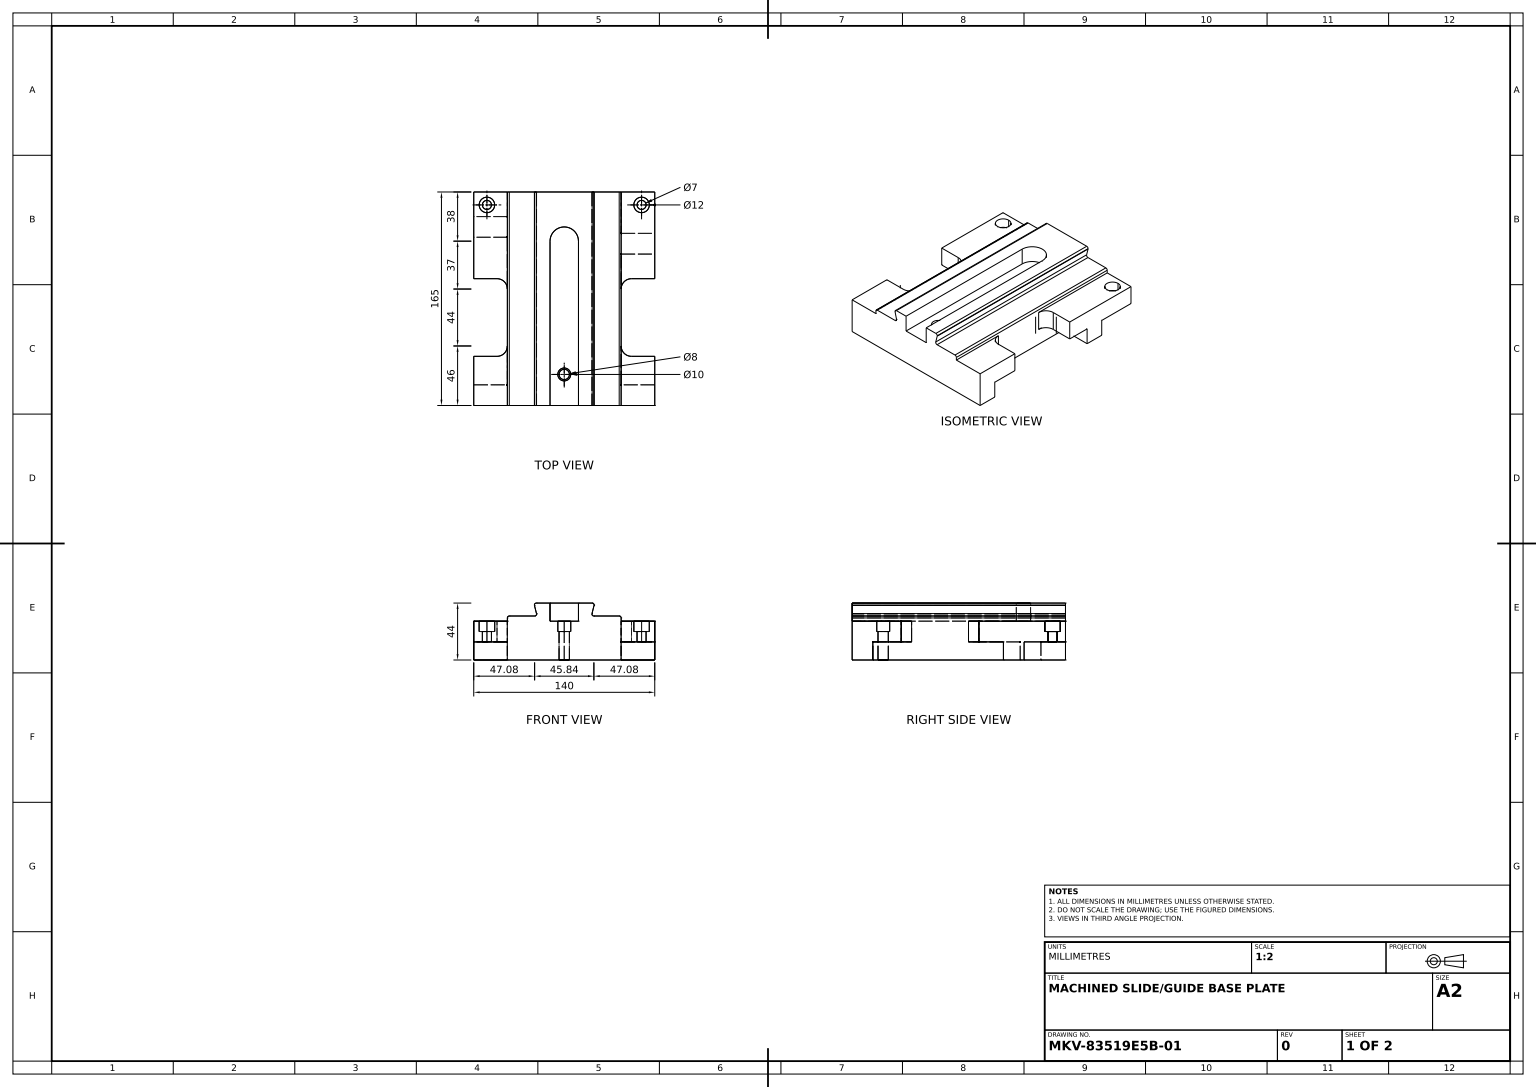
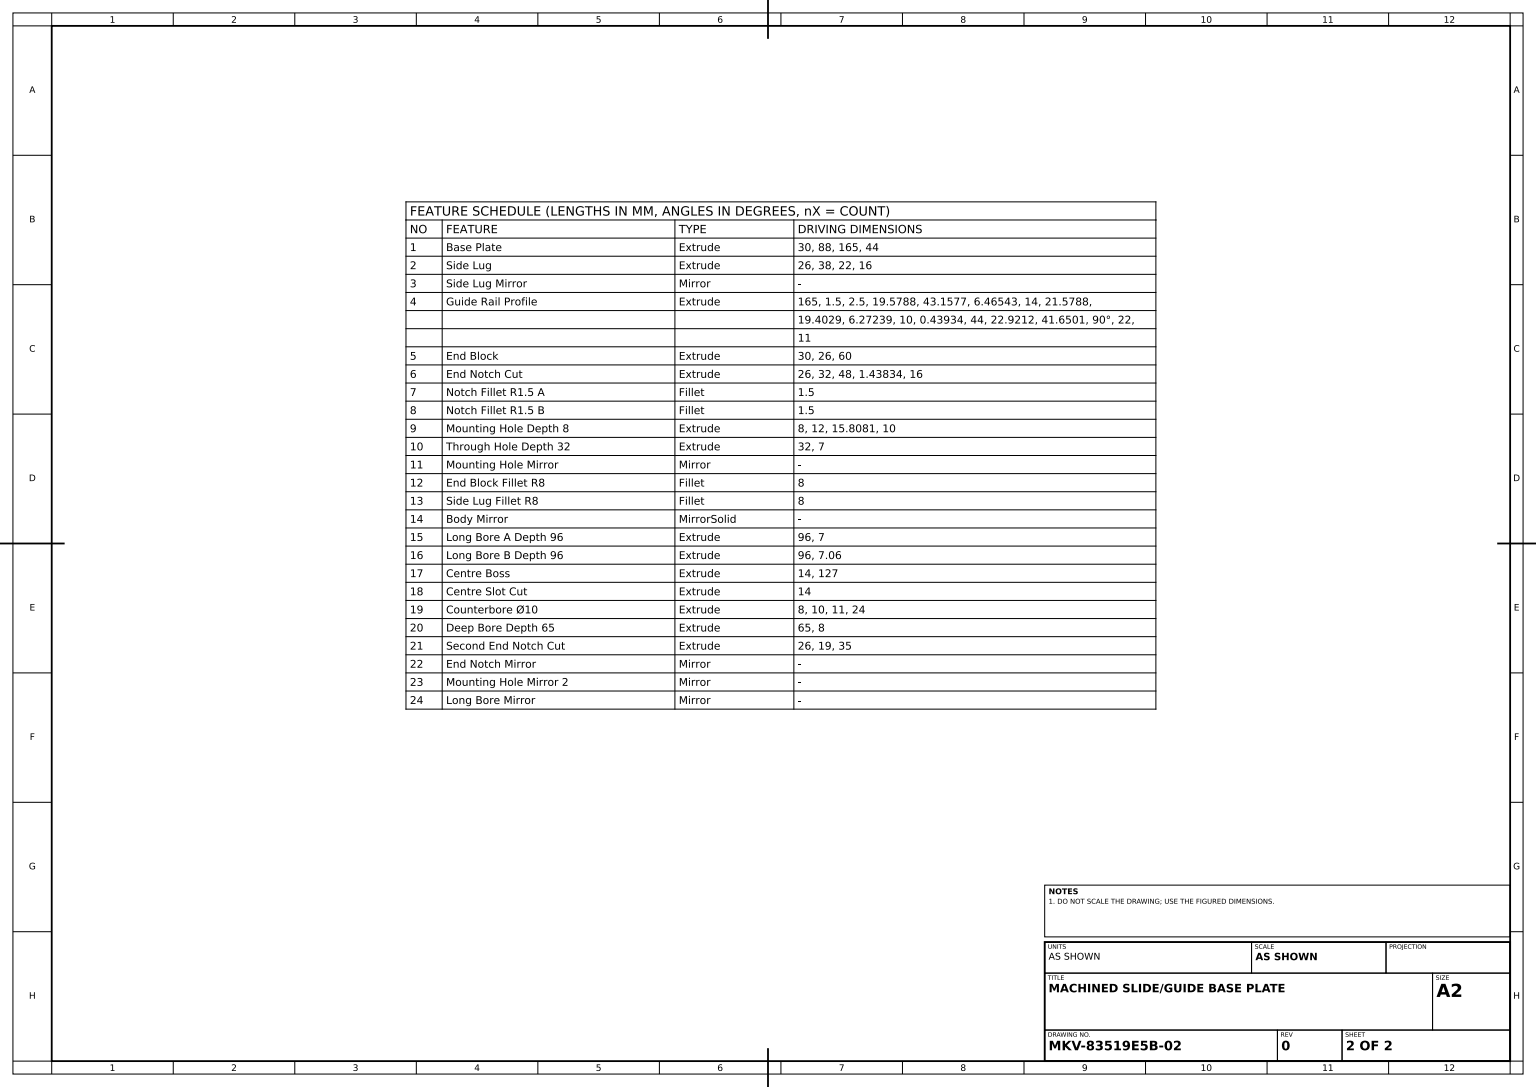
solid
v1 (-59.808083,-16,-76)
v2 (-59.808083,-16,-69)
e1 v1 v2 CIRCLE(AX(P(-59.808083,-16,-72.5),D(0,-1,0),D(0,0,1)),3.5)
e2 v2 v1 CIRCLE(AX(P(-59.808083,-16,-72.5),D(0,-1,0),D(0,0,1)),3.5)
v3 (-44,-16,-63.5)
v4 (-44,-16,-82.5)
e3 v3 v4 LINE
v5 (-70,-16,-63.5)
e4 v3 v5 LINE
v6 (-70,-16,-82.5)
e5 v5 v6 LINE
e6 v4 v6 LINE
face PLANE(AX(P(-44,-16,0),D(0,1,0),D(0,0,1))) rev [-e1 -e2] [-e3 e4 e5 -e6]
v7 (59.808083,-16,-76)
v8 (59.808083,-16,-69)
e7 v7 v8 CIRCLE(AX(P(59.808083,-16,-72.5),D(0,1,0),D(0,0,-1)),3.5)
e8 v8 v7 CIRCLE(AX(P(59.808083,-16,-72.5),D(0,1,0),D(0,0,-1)),3.5)
v9 (44,-16,-82.5)
v10 (70,-16,-82.5)
e9 v9 v10 LINE
v11 (70,-16,-50.5)
e10 v11 v10 LINE
v12 (44,-16,-50.5)
e11 v12 v11 LINE
e12 v12 v9 LINE
face PLANE(AX(P(44,-16,0),D(0,-1,0),D(0,0,-1))) [e7 e8] [e9 -e10 -e11 e12]
v13 (0,-8,62.5)
v14 (0,-8,54.5)
e13 v13 v14 CIRCLE(AX(P(0,-8,58.5),D(0,1,0),D(0,0,1)),4)
e14 v14 v13 CIRCLE(AX(P(0,-8,58.5),D(0,1,0),D(0,0,1)),4)
v15 (0,-8,53.5)
v16 (0,-8,63.5)
e15 v15 v16 CIRCLE(AX(P(0,-8,58.5),D(0,1,0),D(0,0,1)),5)
e16 v16 v15 CIRCLE(AX(P(0,-8,58.5),D(0,1,0),D(0,0,1)),5)
face PLANE(AX(P(0,-8,58.5),D(0,1,0),D(0,0,1))) [-e13 -e14] [e15 e16]
v17 (-70,0,82.5)
v18 (-70,-30,82.5)
e17 v17 v18 LINE
v19 (-70,0,44.5)
e18 v19 v17 LINE
v20 (-70,-16,44.5)
e19 v20 v19 LINE
v21 (-70,-16,66.5)
e20 v21 v20 LINE
v22 (-70,-30,66.5)
e21 v22 v21 LINE
e22 v18 v22 LINE
face PLANE(AX(P(-70,0,0),D(-1,0,0),D(0,0,-1))) [-e17 -e18 -e19 -e20 -e21 -e22]
v23 (23.078835,12.5,-82.5)
v24 (23.034049,12.136197,-82.5)
e23 v23 v24 CIRCLE(AX(P(21.578835,12.5,-82.5),D(0,0,-1),D(1,0,0)),1.5)
v25 (23.078835,12.5,82.5)
e24 v23 v25 LINE
v26 (23.034049,12.136197,82.5)
e25 v25 v26 CIRCLE(AX(P(21.578835,12.5,82.5),D(0,0,-1),D(1,0,0)),1.5)
e26 v24 v26 LINE
face CYL(AX(P(21.578835,12.5,-82.5),D(0,0,1),D(1,0,0)),1.5) [-e23 e24 e25 -e26]
v27 (0,-30,54.5)
e27 v27 v14 LINE
v28 (0,-30,62.5)
e28 v27 v28 CIRCLE(AX(P(0,-30,58.5),D(0,-1,0),D(0,0,-1)),4)
e29 v28 v13 LINE
face CYL(AX(P(0,-73,58.5),D(0,1,0),D(0,0,1)),4) rev [-e27 e28 e29 e13]
v29 (-21.578835,14,-82.5)
v30 (-23.034049,12.136197,-82.5)
e30 v29 v30 CIRCLE(AX(P(-21.578835,12.5,-82.5),D(0,0,1),D(1,0,0)),1.5)
v31 (-23.034049,12.136197,82.5)
e31 v30 v31 LINE
v32 (-21.578835,14,82.5)
e32 v32 v31 CIRCLE(AX(P(-21.578835,12.5,82.5),D(0,0,1),D(1,0,0)),1.5)
e33 v29 v32 LINE
face CYL(AX(P(-21.578835,12.5,-82.5),D(0,0,1),D(1,0,0)),1.5) [e30 e31 -e32 -e33]
v33 (-70,-30,-47.5)
v34 (-70,-16,-47.5)
e34 v33 v34 LINE
v35 (-44,-30,-47.5)
e35 v35 v33 LINE
v36 (-44,-16,-47.5)
e36 v35 v36 LINE
e37 v36 v34 LINE
face PLANE(AX(P(-44,0,-47.5),D(0,0,1),D(1,0,0))) [-e34 -e35 e36 e37]
v37 (70,0,-15.5)
v38 (52,0,-15.5)
e38 v37 v38 LINE
v39 (52,-16,-15.5)
e39 v39 v38 LINE
v40 (70,-16,-15.5)
e40 v39 v40 LINE
e41 v40 v37 LINE
face PLANE(AX(P(44,-30,-15.5),D(0,0,-1),D(-1,0,0))) rev [e38 -e39 e40 e41]
v41 (-44,0,-7.5)
v42 (-52,0,-15.5)
e42 v41 v42 CIRCLE(AX(P(-52,0,-7.5),D(0,1,0),D(0,0,1)),8)
v43 (-52,-16,-15.5)
e43 v43 v42 LINE
v44 (-44,-16,-7.5)
e44 v43 v44 CIRCLE(AX(P(-52,-16,-7.5),D(0,-1,0),D(0,0,-1)),8)
e45 v41 v44 LINE
face CYL(AX(P(-52,-30,-7.5),D(0,-1,0),D(0,0,-1)),8) rev [e42 -e43 e44 -e45]
v45 (44,0,-7.5)
e46 v45 v38 CIRCLE(AX(P(52,0,-7.5),D(0,-1,0),D(0,0,1)),8)
v46 (44,-16,-7.5)
e47 v45 v46 LINE
e48 v39 v46 CIRCLE(AX(P(52,-16,-7.5),D(0,1,0),D(0,0,-1)),8)
face CYL(AX(P(52,-30,-7.5),D(0,-1,0),D(0,0,-1)),8) rev [-e46 e47 -e48 e39]
v47 (-21.465951,5.863803,-82.5)
e49 v47 v30 LINE
v48 (-21.465951,5.863803,82.5)
e50 v47 v48 LINE
e51 v48 v31 LINE
face PLANE(AX(P(-18.823529,-4.705882,-82.5),D(0.9701425,0.242535625,0),D(-0.242535625,0.9701425,0))) rev [-e31 -e49 e50 e51]
v49 (-44,2.500001,82.5)
v50 (-42.500001,4,82.5)
e52 v49 v50 CIRCLE(AX(P(-42.5,2.5,82.5),D(0,0,-1),D(1,0,0)),1.5)
v51 (-42.500001,4,-82.5)
e53 v51 v50 LINE
v52 (-44,2.500001,-82.5)
e54 v52 v51 CIRCLE(AX(P(-42.5,2.5,-82.5),D(0,0,-1),D(1,0,0)),1.5)
e55 v52 v49 LINE
face CYL(AX(P(-42.5,2.5,-82.5),D(0,0,1),D(1,0,0)),1.5) [e52 -e53 -e54 e55]
v53 (70,-30,66.5)
v54 (70,-16,66.5)
e56 v53 v54 LINE
v55 (44,-30,66.5)
e57 v53 v55 LINE
v56 (44,-16,66.5)
e58 v55 v56 LINE
e59 v54 v56 LINE
face PLANE(AX(P(70,-30,66.5),D(0,0,1),D(1,0,0))) rev [-e56 e57 e58 -e59]
v57 (-59.808083,-8,-78.5)
v58 (-59.808083,-8,-66.5)
e60 v57 v58 CIRCLE(AX(P(-59.808083,-8,-72.5),D(0,1,0),D(0,0,1)),6)
e61 v58 v57 CIRCLE(AX(P(-59.808083,-8,-72.5),D(0,1,0),D(0,0,1)),6)
v59 (-59.808083,-8,-76)
v60 (-59.808083,-8,-69)
e62 v59 v60 CIRCLE(AX(P(-59.808083,-8,-72.5),D(0,1,0),D(0,0,1)),3.5)
e63 v60 v59 CIRCLE(AX(P(-59.808083,-8,-72.5),D(0,1,0),D(0,0,1)),3.5)
face PLANE(AX(P(-59.808083,-8,-72.5),D(0,1,0),D(0,0,1))) [e60 e61] [-e62 -e63]
v61 (44,2.5,-82.5)
v62 (44,2.5,82.5)
e64 v61 v62 LINE
v63 (44,0,82.5)
e65 v63 v62 LINE
v64 (44,0,36.5)
e66 v64 v63 LINE
v65 (44,-16,36.5)
e67 v65 v64 LINE
e68 v56 v65 LINE
v66 (44,-30,-34.5)
e69 v55 v66 LINE
v67 (44,-16,-34.5)
e70 v67 v66 LINE
e71 v67 v46 LINE
v68 (44,0,-82.5)
e72 v45 v68 LINE
e73 v68 v61 LINE
face PLANE(AX(P(44,-30,-82.5),D(1,0,0),D(0,0,-1))) [e64 -e65 -e66 -e67 -e68 -e58 e69 -e70 e71 -e47 e72 e73]
e74 v1 v59 LINE
e75 v2 v60 LINE
face CYL(AX(P(-59.808083,-104,-72.5),D(0,1,0),D(0,0,1)),3.5) rev [e74 e62 -e75 e2]
v69 (42.5,4,-82.5)
v70 (42.5,4,82.5)
e76 v69 v70 LINE
v71 (22.921165,4,-82.5)
e77 v69 v71 LINE
v72 (22.921165,4,82.5)
e78 v71 v72 LINE
e79 v70 v72 LINE
face PLANE(AX(P(0,4,-82.5),D(0,1,0),D(-1,0,0))) [-e76 e77 e78 -e79]
v73 (44,-30,-82.5)
v74 (44,-30,-50.5)
e80 v73 v74 LINE
e81 v9 v73 LINE
e82 v74 v12 LINE
face PLANE(AX(P(44,0,0),D(1,0,0),D(0,0,1))) [-e80 -e81 -e12 -e82]
v75 (52,-16,44.5)
e83 v65 v75 CIRCLE(AX(P(52,-16,36.5),D(0,1,0),D(0,0,-1)),8)
v76 (70,-16,44.5)
e84 v76 v75 LINE
e85 v54 v76 LINE
face PLANE(AX(P(70,-16,66.5),D(0,1,0),D(0,0,1))) rev [e83 -e84 -e85 e59 e68]
v77 (11,14,-44.5)
v78 (-11,14,-44.5)
e86 v77 v78 CIRCLE(AX(P(0,14,-44.5),D(0,1,0),D(-1,0,0)),11)
v79 (-11,0,-44.5)
e87 v79 v78 LINE
v80 (11,0,-44.5)
e88 v80 v79 CIRCLE(AX(P(0,0,-44.5),D(0,1,0),D(-1,0,0)),11)
e89 v80 v77 LINE
face CYL(AX(P(0,0,-44.5),D(0,1,0),D(-1,0,0)),11) rev [e86 -e87 -e88 e89]
v81 (-70,0,-82.5)
v82 (-70,0,-15.5)
e90 v81 v82 LINE
e91 v6 v81 LINE
v83 (-70,-30,-63.5)
e92 v5 v83 LINE
e93 v83 v33 LINE
v84 (-70,-16,-15.5)
e94 v34 v84 LINE
e95 v84 v82 LINE
face PLANE(AX(P(-70,-30,-15.5),D(-1,0,0),D(0,0,1))) [-e90 -e91 -e5 e92 e93 e34 e94 e95]
v85 (21.578835,14,-82.5)
e96 v85 v23 CIRCLE(AX(P(21.578835,12.5,-82.5),D(0,0,-1),D(1,0,0)),1.5)
v86 (21.578835,14,82.5)
e97 v85 v86 LINE
e98 v86 v25 CIRCLE(AX(P(21.578835,12.5,82.5),D(0,0,-1),D(1,0,0)),1.5)
face CYL(AX(P(21.578835,12.5,-82.5),D(0,0,1),D(1,0,0)),1.5) [-e96 e97 e98 -e24]
e99 v28 v27 CIRCLE(AX(P(0,-30,58.5),D(0,-1,0),D(0,0,-1)),4)
v87 (-44,-30,-82.5)
e100 v73 v87 LINE
v88 (70,-30,-50.5)
e101 v74 v88 LINE
v89 (70,-30,-34.5)
e102 v88 v89 LINE
e103 v66 v89 LINE
v90 (70,-30,82.5)
e104 v90 v53 LINE
e105 v18 v90 LINE
v91 (-44,-30,66.5)
e106 v22 v91 LINE
e107 v35 v91 LINE
v92 (-44,-30,-63.5)
e108 v92 v83 LINE
e109 v87 v92 LINE
face PLANE(AX(P(0,-30,0),D(0,-1,0),D(0,0,-1))) [-e99 -e28] [-e100 e80 e101 e102 -e103 -e69 -e57 -e104 -e105 e22 e106 -e107 e35 -e93 -e108 -e109]
v93 (59.808083,0,-78.5)
v94 (59.808083,0,-66.5)
e110 v93 v94 CIRCLE(AX(P(59.808083,0,-72.5),D(0,-1,0),D(0,0,1)),6)
v95 (59.808083,-8,-78.5)
e111 v95 v93 LINE
v96 (59.808083,-8,-66.5)
e112 v95 v96 CIRCLE(AX(P(59.808083,-8,-72.5),D(0,-1,0),D(0,0,1)),6)
e113 v96 v94 LINE
face CYL(AX(P(59.808083,-8,-72.5),D(0,1,0),D(0,0,1)),6) rev [-e110 -e111 e112 e113]
e114 v61 v69 CIRCLE(AX(P(42.5,2.5,-82.5),D(0,0,1),D(1,0,0)),1.5)
v97 (70,0,-82.5)
e115 v68 v97 LINE
e116 v10 v97 LINE
e117 v4 v87 LINE
v98 (-44,0,-82.5)
e118 v98 v81 LINE
e119 v98 v52 LINE
v99 (-22.921165,4,-82.5)
e120 v51 v99 LINE
v100 (-21.421165,5.5,-82.5)
e121 v99 v100 CIRCLE(AX(P(-22.921165,5.5,-82.5),D(0,0,1),D(1,0,0)),1.5)
e122 v100 v47 CIRCLE(AX(P(-22.921165,5.5,-82.5),D(0,0,1),D(1,0,0)),1.5)
e123 v29 v85 LINE
v101 (21.465951,5.863803,-82.5)
e124 v101 v24 LINE
e125 v71 v101 CIRCLE(AX(P(22.921165,5.5,-82.5),D(0,0,-1),D(1,0,0)),1.5)
face PLANE(AX(P(-44,-30,-82.5),D(0,0,-1),D(-1,0,0))) [-e77 -e114 -e73 e115 -e116 -e9 e81 e100 -e117 e6 e91 -e118 e119 e54 e120 e121 e122 e49 -e30 e123 e96 e23 -e124 -e125]
v102 (-52,0,44.5)
e126 v19 v102 LINE
v103 (-52,-16,44.5)
e127 v102 v103 LINE
e128 v20 v103 LINE
face PLANE(AX(P(-70,0,44.5),D(0,0,-1),D(0,1,0))) [e126 e127 -e128 e19]
v104 (-44,-16,36.5)
e129 v104 v103 CIRCLE(AX(P(-52,-16,36.5),D(0,-1,0),D(0,0,-1)),8)
v105 (-44,-16,66.5)
e130 v105 v104 LINE
e131 v21 v105 LINE
face PLANE(AX(P(-70,-16,66.5),D(0,-1,0),D(0,0,-1))) [-e129 -e130 -e131 e20 e128]
e132 v96 v95 CIRCLE(AX(P(59.808083,-8,-72.5),D(0,-1,0),D(0,0,1)),6)
v106 (59.808083,-8,-76)
v107 (59.808083,-8,-69)
e133 v106 v107 CIRCLE(AX(P(59.808083,-8,-72.5),D(0,-1,0),D(0,0,1)),3.5)
e134 v107 v106 CIRCLE(AX(P(59.808083,-8,-72.5),D(0,-1,0),D(0,0,1)),3.5)
face PLANE(AX(P(59.808083,-8,-72.5),D(0,1,0),D(0,0,1))) [-e112 -e132] [e133 e134]
v108 (70,-16,-34.5)
e135 v108 v89 LINE
e136 v67 v108 LINE
face PLANE(AX(P(44,0,-34.5),D(0,0,1),D(1,0,0))) [e103 -e135 -e136 e70]
v109 (-44,0,36.5)
e137 v102 v109 CIRCLE(AX(P(-52,0,36.5),D(0,1,0),D(0,0,-1)),8)
v110 (-44,0,82.5)
e138 v17 v110 LINE
e139 v109 v110 LINE
face PLANE(AX(P(0,0,0),D(0,-1,0),D(0,0,-1))) rev [-e137 -e126 e18 e138 -e139]
v111 (-11,0,82.5)
e140 v79 v111 LINE
v112 (11,0,82.5)
e141 v111 v112 LINE
e142 v80 v112 LINE
v113 (0,0,63.5)
v114 (0,0,53.5)
e143 v113 v114 CIRCLE(AX(P(0,0,58.5),D(0,1,0),D(0,0,1)),5)
e144 v114 v113 CIRCLE(AX(P(0,0,58.5),D(0,1,0),D(0,0,1)),5)
face PLANE(AX(P(0,0,0),D(0,-1,0),D(0,0,-1))) rev [e140 e141 -e142 e88] [-e143 -e144]
e145 v3 v92 LINE
face PLANE(AX(P(-44,0,0),D(-1,0,0),D(0,0,1))) [-e145 e3 e117 e109]
e146 v88 v11 LINE
e147 v97 v37 LINE
e148 v108 v40 LINE
face PLANE(AX(P(70,-30,-15.5),D(-1,0,0),D(0,0,1))) rev [e135 -e102 e146 e10 e116 e147 -e41 -e148]
e149 v15 v114 LINE
e150 v16 v113 LINE
face CYL(AX(P(0,-8,58.5),D(0,1,0),D(0,0,1)),5) rev [-e149 -e16 e150 e143]
v115 (-11,14,82.5)
e151 v32 v115 LINE
e152 v78 v115 LINE
v116 (11,14,82.5)
e153 v77 v116 LINE
e154 v116 v86 LINE
face PLANE(AX(P(0,14,-82.5),D(0,-1,0),D(1,0,0))) rev [-e97 -e123 e33 e151 -e152 -e86 e153 e154]
e155 v116 v112 LINE
face PLANE(AX(P(11,0,-82.5),D(-1,0,0),D(0,0,1))) [-e155 -e153 -e89 e142]
face CYL(AX(P(-59.808083,-104,-72.5),D(0,1,0),D(0,0,1)),3.5) rev [e63 -e74 e1 e75]
e156 v94 v93 CIRCLE(AX(P(59.808083,0,-72.5),D(0,-1,0),D(0,0,1)),6)
face PLANE(AX(P(0,0,0),D(0,1,0),D(0,0,1))) [-e147 -e115 -e72 e46 -e38] [e156 e110]
v117 (-21.421165,5.5,82.5)
e157 v100 v117 LINE
e158 v117 v48 CIRCLE(AX(P(-22.921165,5.5,82.5),D(0,0,1),D(1,0,0)),1.5)
face CYL(AX(P(-22.921165,5.5,-82.5),D(0,0,1),D(1,0,0)),1.5) rev [-e50 -e122 e157 e158]
e159 v111 v115 LINE
face PLANE(AX(P(-11,0,-82.5),D(1,0,0),D(0,1,0))) [e87 e152 -e159 -e140]
v118 (-59.808083,0,-66.5)
v119 (-59.808083,0,-78.5)
e160 v118 v119 CIRCLE(AX(P(-59.808083,0,-72.5),D(0,1,0),D(0,0,1)),6)
e161 v57 v119 LINE
e162 v58 v118 LINE
face CYL(AX(P(-59.808083,-8,-72.5),D(0,1,0),D(0,0,1)),6) rev [e160 -e161 -e61 e162]
face CYL(AX(P(0,-73,58.5),D(0,1,0),D(0,0,1)),4) rev [e99 e27 e14 -e29]
e163 v43 v84 LINE
e164 v36 v44 LINE
face PLANE(AX(P(-44,-16,0),D(0,-1,0),D(0,0,-1))) [e163 -e94 -e37 e164 -e44]
v120 (70,0,44.5)
v121 (70,0,82.5)
e165 v120 v121 LINE
v122 (52,0,44.5)
e166 v120 v122 LINE
e167 v122 v64 CIRCLE(AX(P(52,0,36.5),D(0,-1,0),D(0,0,-1)),8)
e168 v63 v121 LINE
face PLANE(AX(P(0,0,0),D(0,-1,0),D(0,0,-1))) rev [-e165 e166 e167 e66 e168]
v123 (21.465951,5.863803,82.5)
e169 v101 v123 LINE
e170 v72 v123 CIRCLE(AX(P(22.921165,5.5,82.5),D(0,0,-1),D(1,0,0)),1.5)
face CYL(AX(P(22.921165,5.5,-82.5),D(0,0,1),D(1,0,0)),1.5) rev [e125 e169 -e170 -e78]
face CYL(AX(P(0,-8,58.5),D(0,1,0),D(0,0,1)),5) rev [e149 e144 -e150 -e15]
e171 v122 v75 LINE
face CYL(AX(P(52,0,36.5),D(0,1,0),D(0,0,1)),8) rev [-e167 e171 -e83 e67]
face CYL(AX(P(59.808083,-8,-72.5),D(0,1,0),D(0,0,1)),6) rev [-e113 e132 e111 -e156]
face PLANE(AX(P(-44,0,-63.5),D(0,0,-1),D(-1,0,0))) [-e4 e145 e108 -e92]
e172 v119 v118 CIRCLE(AX(P(-59.808083,0,-72.5),D(0,1,0),D(0,0,1)),6)
e173 v82 v42 LINE
e174 v41 v98 LINE
face PLANE(AX(P(0,0,0),D(0,1,0),D(0,0,1))) [-e172 -e160] [e118 e90 e173 -e42 e174]
e175 v62 v70 CIRCLE(AX(P(42.5,2.5,82.5),D(0,0,1),D(1,0,0)),1.5)
e176 v123 v26 LINE
v124 (-22.921165,4,82.5)
e177 v124 v117 CIRCLE(AX(P(-22.921165,5.5,82.5),D(0,0,1),D(1,0,0)),1.5)
e178 v50 v124 LINE
e179 v110 v49 LINE
e180 v121 v90 LINE
face PLANE(AX(P(44,-30,82.5),D(0,0,1),D(1,0,0))) [e65 e175 e79 e170 e176 -e25 -e98 -e154 e155 -e141 e159 -e151 e32 -e51 -e158 -e177 -e178 -e52 -e179 -e138 e17 e105 -e180 -e168]
e181 v76 v120 LINE
face PLANE(AX(P(70,0,44.5),D(0,0,1),D(0,-1,0))) rev [e84 -e171 -e166 -e181]
e182 v8 v107 LINE
e183 v7 v106 LINE
face CYL(AX(P(59.808083,-104,-72.5),D(0,1,0),D(0,0,1)),3.5) rev [-e8 e182 -e133 -e183]
e184 v99 v124 LINE
face CYL(AX(P(-22.921165,5.5,-82.5),D(0,0,1),D(1,0,0)),1.5) rev [e184 e177 -e157 -e121]
e185 v91 v105 LINE
face PLANE(AX(P(-70,-30,66.5),D(0,0,-1),D(-1,0,0))) [e21 e131 -e185 -e106]
e186 v104 v109 LINE
face PLANE(AX(P(-44,-30,82.5),D(-1,0,0),D(0,0,1))) [-e55 -e119 -e174 e45 -e164 -e36 e107 e185 e130 e186 e139 e179]
face CYL(AX(P(59.808083,-104,-72.5),D(0,1,0),D(0,0,1)),3.5) rev [e183 -e134 -e182 -e7]
face PLANE(AX(P(70,0,0),D(1,0,0),D(0,0,-1))) [e85 e181 e165 e180 e104 e56]
face CYL(AX(P(-52,0,36.5),D(0,1,0),D(0,0,1)),8) rev [e129 -e127 e137 -e186]
face PLANE(AX(P(0,4,-82.5),D(0,-1,0),D(0,0,-1))) rev [-e184 -e120 e53 e178]
face PLANE(AX(P(44,0,-50.5),D(0,0,-1),D(-1,0,0))) [e82 e11 -e146 -e101]
face CYL(AX(P(-59.808083,-8,-72.5),D(0,1,0),D(0,0,1)),6) rev [e172 -e162 -e60 e161]
face CYL(AX(P(42.5,2.5,-82.5),D(0,0,1),D(1,0,0)),1.5) [e114 e76 -e175 -e64]
face PLANE(AX(P(18.823529,-4.705882,-82.5),D(0.9701425,-0.242535625,0),D(0.242535625,0.9701425,0))) [-e176 -e169 e124 e26]
face PLANE(AX(P(44,-16,0),D(0,-1,0),D(0,0,-1))) [-e71 e136 e148 -e40 e48]
face PLANE(AX(P(-44,-30,-15.5),D(0,0,1),D(1,0,0))) [-e95 -e163 e43 -e173]
